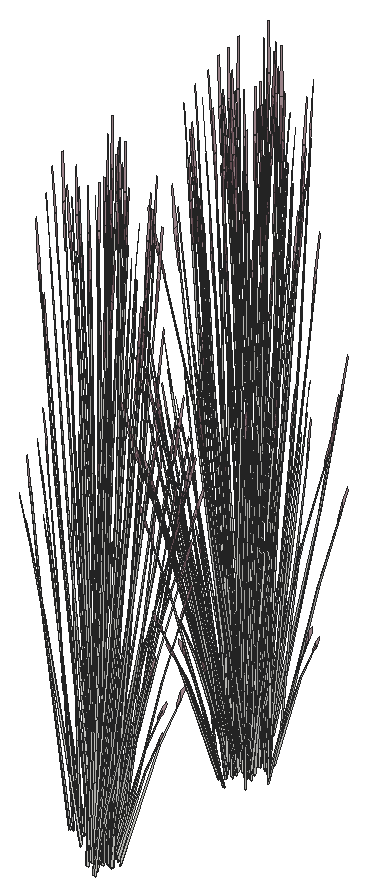
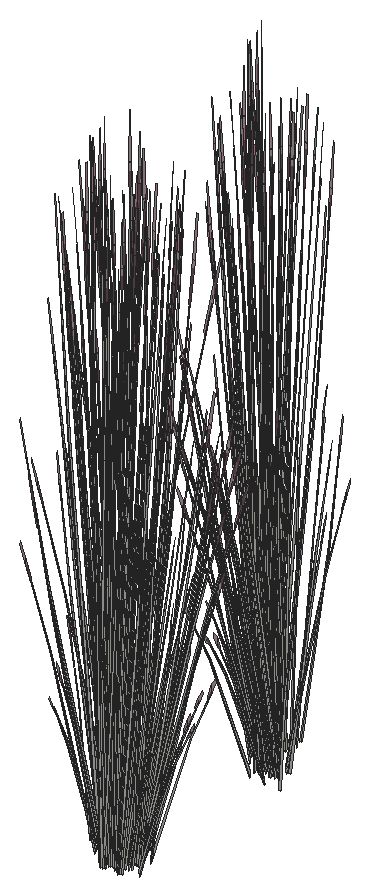
# SketchUp Ruby script. Lengths in inches.
U = 1.inch
M = Sketchup.active_model
def pt(a) = Geom::Point3d.new(a.map { |v| v * U })
def face(e, loops, mat)
  f = e.add_face(loops[0].map { |a| pt(a) })
  loops[1..].each { |l| e.add_face(l.map { |a| pt(a) }).erase! }
  f.material = f.back_material = mat if mat
  f
end
# faces: each face lists its corners as indices into pts; further lists are holes
def faces(e, pts, list, mat = nil) = list.each { |f| face(e, (f[0].is_a?(Array) ? f : [f]).map { |l| l.map { |i| pts[i] } }, mat) }
# xy, xz, yz: faces in a plane at the given z, y or x. An outline is a flat list of corners, or four numbers for a rectangle; further outlines are holes
def ring(l) = l.size == 4 ? [[l[0], l[1]], [l[2], l[1]], [l[2], l[3]], [l[0], l[3]]] : l.each_slice(2).to_a
def flat(e, list, mat, &to3) = list.each { |f| face(e, (f[0].is_a?(Array) ? f : [f]).map { |l| ring(l).map { |u, v| to3.(u, v) } }, mat) }
def xy(e, z, list, mat = nil) = flat(e, list, mat) { |x, y| [x, y, z] }
def xz(e, y, list, mat = nil) = flat(e, list, mat) { |x, z| [x, y, z] }
def yz(e, x, list, mat = nil) = flat(e, list, mat) { |y, z| [x, y, z] }
def lines(e, pts, list) = list.each { |a, b| e.add_line(pt(pts[a]), pt(pts[b])) }
# prism: a flat outline (further loops are holes) pulled along v
def prism(e, loops, v, mat = nil)
  f = face(e, loops, mat); d = Geom::Vector3d.new(v.map { |x| x * U })
  f.pushpull(f.normal.samedirection?(d) ? d.length : -d.length)
end
def box(e, o, s, mat = nil) = prism(e, [[o, [o[0] + s[0], o[1], o[2]], [o[0] + s[0], o[1] + s[1], o[2]], [o[0], o[1] + s[1], o[2]]]], [0, 0, s[2]], mat)
def at(x, y, z, deg = 0) = Geom::Transformation.translation(pt([x, y, z])) * Geom::Transformation.rotation(ORIGIN, Z_AXIS, deg.degrees)
def axes(o, x, y, z) = Geom::Transformation.new([*x, 0, *y, 0, *z, 0, *pt(o).to_a, 1])
def part(name) = M.definitions.add(name)
# library, detail: a bought-in or finely detailed component or shape, given as its bounding box
def library(name, o, s) = part(name).tap { |d| box(d.entities, o, s) }
def detail(e, o, s) = box(e.add_group.entities, o, s)
def put(e, d, t, mat = nil) = e.add_instance(d, t).tap { |i| i.material = mat if mat }
def group(e, t, mat = nil) = e.add_group.tap { |g| g.transformation = t; g.material = mat if mat }.entities
root = M.entities
M.materials.add("LightPink_Translucent").color = [144, 107, 117]
M.materials["LightPink_Translucent"].alpha = 0.75
c1 = part("blade")
p = [[2.15,0.21,22],[0,0.17,0],[0.09,0.45,0],[2.18,0.31,22],[2.29,0.31,22],[0.38,0.45,0],
  [2.48,0.24,33],[2.49,0.24,33],[2.48,0.22,33]]
faces(c1.entities,p,[[0,1,2,3],[4,5,2,3],[6,3,4,7],[8,0,3,6]])
c2 = part("seeds")
p = [[0.3,-0.1,1.38],[-0.01,-0.03,1.59],[-0.01,-0.03,0.03],[0.14,-0.07,-0.07],[0.29,-0.03,3],[0.15,0.01,3.11]]
faces(c2.entities,p,[[0,1,2,3],[1,0,4,5]],"LightPink_Translucent")
c3 = part("blade with seeds")
put(c3.entities,c1,at(0,0,0))
put(c3.entities,c2,axes([2.4,0.25,30.99],[1.5799,-0.05474,1.17369],[-0.12525,1.92788,0.29478],[-0.07173,-0.02425,1.56792]))
put(root,c3,axes([402.25,60.02,2.72],[-0.21202,-0.39143,0.44739],[0.32115,-0.27564,-0.21531],[0.06861,0.04843,1.43643]))
put(root,c3,axes([401.15,61.81,2.03],[-0.08291,-0.40636,-0.30978],[0.32928,-0.11539,0.30978],[-0.06638,-0.04686,1.38974]))
put(root,c3,axes([401.58,61.78,2.47],[0.37926,-0.12378,0.17642],[0.09365,0.46065,0.35086],[-0.03382,-0.06712,1.60407]))
put(root,c3,axes([402.36,60.04,2.67],[0.35635,-0.30962,-0.29095],[0.23697,0.43749,-0.50002],[0.08792,0.04443,1.59708]))
put(root,c3,axes([403.78,60.86,4.53],[0.29332,0.1301,-0.35414],[-0.08555,0.37955,0.4572],[0.11809,-0.0348,0.87481]))
put(root,c3,axes([401.0625,61.98,2.02],[-0.33032,-0.23318,-0.49651],[0.19744,-0.41812,0],[-0.07523,-0.05311,1.57504]))
put(root,c3,axes([403.26,59.22,2.02],[0.33032,0.23318,-0.49651],[-0.19744,0.41812,0],[0.07523,0.05311,1.57504]))
put(root,c3,axes([400.33,60.25,4.53],[-0.29332,-0.1301,-0.35414],[0.08555,-0.37955,0.4572],[-0.11809,0.0348,0.87481]))
put(root,c3,axes([402.63,60.55,2.21],[0.39487,0,0],[0,0.48281,0],[0,0,1.78407]))
put(root,c3,axes([401.96,61.16,2.67],[-0.35635,0.30962,-0.29095],[-0.23697,-0.43749,-0.50002],[-0.08792,-0.04443,1.59708]))
put(root,c3,axes([402.74,59.42,2.47],[-0.37926,0.12378,0.17642],[-0.09365,-0.46065,0.35086],[0.03382,0.06712,1.60407]))
put(root,c3,axes([402.98,60.39,3.875],[-0.14639,0.01056,1.71376],[0.09712,-0.45778,0.13857],[0.20862,0.02831,0.73262]))
put(root,c3,axes([403.17,59.39,2.03],[0.08291,0.40636,-0.30978],[-0.32928,0.11539,0.30978],[0.06638,0.04686,1.38974]))
put(root,c3,axes([402.5,60.3,2.38],[-0.44609,-0.09826,0.49198],[0.09078,-0.55493,0.19306],[0.06519,0.05359,1.70813]))
put(root,c3,axes([402.15,61.67,2.2],[-0.11516,-0.40207,0],[0.32884,-0.1408,0],[0,0,1.54371]))
put(root,c3,axes([401.93,61.29,2.62],[-0.06809,0.4162,0.1448],[-0.33266,-0.07225,-0.41347],[-0.06054,-0.04274,1.26744]))
put(root,c3,axes([402.58,61.62,2.18],[0.37054,-0.15823,-0.19198],[0.1302,0.45581,0.00008],[0.0409,-0.01749,1.73897]))
put(root,c3,axes([402.71,61.81,2.47],[0.10196,-0.46348,0.17642],[0.3731,0.13116,0.35086],[-0.06445,0.00226,1.60407]))
put(root,c3,axes([402.62,60.76,2.21],[0.24637,0.30123,0],[-0.24637,0.30123,0],[0,0,1.69266]))
put(root,c3,axes([401.22,60.19,3.34],[0.10032,-0.06746,1.77064],[0.0346,0.47103,0.13857],[-0.2173,0.0625,0.63284]))
put(root,c3,axes([403.29,60.625,2.47],[-0.2773,-0.3397,0.17642],[0.27945,-0.32949,0.35086],[-0.03063,0.06937,1.60407]))
put(root,c3,axes([402.78,60.11,2.06],[0.36714,0.07646,-0.62353],[-0.07747,0.47163,-0.16365],[0.10956,0.05715,1.37633]))
put(root,c3,axes([404.4,60.9375,2.77],[-0.21807,0.07699,1.1486],[0.10265,-0.31819,0.84392],[0.11568,0.02177,0.25299]))
put(root,c3,axes([402.07,61.86,2.2],[-0.35581,-0.20937,0],[0.17124,-0.43505,0],[0,0,1.62707]))
put(root,c3,axes([402.36,61.3,2.46],[-0.34464,-0.37536,-0.25192],[0.29,-0.42149,0.5513],[-0.0928,0.04391,1.68216]))
put(root,c3,axes([401.45,62.02,2.48],[0.33032,0.23318,0.49651],[-0.19744,0.41812,0],[-0.07523,-0.05311,1.57504]))
put(root,c3,axes([402.62,60.4,2.72],[0.17124,-0.42022,0.44739],[0.35581,0.20224,-0.21531],[0,0.09687,1.43643]))
put(root,c3,axes([402.55,60.64,2.29],[0,0.53934,-0.05637],[-0.44133,0,0],[0,0.01695,1.79368]))
put(root,c3,axes([400.53,60.45,4.68],[-0.09562,0.42421,-0.51099],[-0.32782,-0.1454,-0.3958],[-0.13199,0.0389,0.97773]))
put(root,c3,axes([402.58,60.26,2.21],[0.21202,0.39143,-0.44739],[-0.32115,0.27564,0.21531],[0.06861,0.04843,1.43643]))
put(root,c3,axes([404.02,61.92,3.93],[-0.06755,-0.39203,-0.03492],[0.31928,-0.09013,-0.15832],[0.06667,0.02485,0.52218]))
put(root,c3,axes([401.26,62.26,2.375],[-0.22066,0.46731,0],[-0.36918,-0.26061,-0.51607],[-0.08408,-0.05936,1.63711]))
put(root,c3,axes([403.52,60.64,2.48],[0,-0.46636,0.49651],[0.39487,0,0],[0,0.10622,1.57504]))
put(root,c3,axes([402.53,60.99,2.72],[0.38326,-0.02879,0.44739],[0.03466,0.47788,-0.21531],[-0.06861,0.04843,1.43643]))
put(root,c3,axes([402.77,60.5,2.62],[0.32884,-0.136,0.1448],[0.11516,0.38837,-0.41347],[0,0.08547,1.26744]))
put(root,c3,axes([402.1875,61.22,2.21],[-0.38326,0.02879,-0.44739],[-0.03466,-0.47788,0.21531],[-0.06861,0.04843,1.43643]))
put(root,c3,axes([403.99,61.45,2.59],[-0.085,-0.1147,1.43002],[0.1106,-0.37943,-0.30754],[0.17198,0.0514,0.61141]))
put(root,c3,axes([402.47,61.86,2.2],[0.35581,0.20937,0],[-0.17124,0.43505,0],[0,0,1.74954]))
put(root,c3,axes([402.61,62.33,2.19],[-0.21791,-0.46895,-0.05142],[0.36918,-0.26061,0.51607],[-0.09097,0.04465,1.6363]))
put(root,c3,axes([402.53,61.19,2.62],[0.26075,0.2802,0.1448],[-0.2175,0.31612,-0.41347],[-0.06054,0.04274,1.26744]))
put(root,c3,axes([400.52,60.67,3.875],[0.12246,-0.09864,1.71376],[0.1031,0.45582,0.13857],[-0.19225,0.10302,0.73262]))
put(root,c3,axes([403.21,61.68,4.98],[0.35281,0.01123,-0.71045],[-0.0237,0.47284,0.08574],[0.14947,0.0499,1.00501]))
put(root,c3,axes([402.8125,62.06,2.48],[0.33032,-0.23318,0.49651],[0.19744,0.41812,0],[-0.07523,0.05311,1.57504]))
put(root,c3,axes([402.34,61.6875,2.29],[0.15345,0.53576,-0.06012],[-0.43845,0.18773,0],[0.00536,0.01871,1.72173]))
put(root,c3,axes([402.51,62.27,2.03],[-0.32928,-0.11539,-0.30978],[0.08291,-0.40636,0.30978],[-0.06638,0.04686,1.38974]))
put(root,c3,axes([400.14,61.44,2.59],[0.12266,0.03828,1.43002],[0.07906,0.39104,-0.30754],[-0.16661,0.0732,0.61141]))
put(root,c3,axes([403.78,60.72,2.375],[0.44133,0,0],[0,0.52122,-0.51607],[0,0.11871,1.63711]))
put(root,c3,axes([403.61,60.99,2.2],[-0.44111,-0.00373,-0.04976],[0,-0.52122,0.49943],[-0.01386,0.11865,1.58352]))
put(root,c3,axes([402.65,60.53,2.67],[0.39748,0.22252,-0.29095],[-0.19139,0.46966,-0.50002],[0.01249,0.11531,1.59708]))
put(root,c3,axes([399.88,62.26,2.77],[0.14709,-0.21136,1.1486],[0.05804,0.3346,0.84392],[-0.1063,0.05991,0.25299]))
put(root,c3,axes([403.42,61.87,4.53],[0.20082,0.29199,-0.35414],[-0.2293,0.2764,0.4572],[0.1165,0.04206,0.87481]))
put(root,c3,axes([403.52,61.0625,2.03],[-0.24637,0.29097,-0.30978],[-0.24637,-0.29097,0.30978],[0,0.09372,1.38974]))
put(root,c3,axes([402.46,61.09,2.67],[0.04113,0.53214,-0.29095],[-0.42835,0.03218,-0.50002],[-0.07543,0.07088,1.59708]))
put(root,c3,axes([402.61,60.88,2.21],[-0.17124,0.42022,-0.44739],[-0.35581,-0.20224,0.21531],[0,0.09687,1.43643]))
put(root,c3,axes([400.43,61.35,4.53],[-0.30722,0.06665,-0.35414],[-0.08112,-0.381,0.4572],[-0.08804,0.10234,0.87481]))
put(root,c3,axes([402.2,61.5,2.06],[-0.23773,0.35053,-0.62353],[-0.29532,-0.31785,-0.16365],[-0.09526,0.08744,1.37633]))
put(root,c3,axes([402.62,62.09,2.33],[0.44186,0.15158,0.30756],[-0.11054,0.54181,-0.36492],[-0.07313,0.06781,1.64885]))
put(root,c3,axes([402.59,62.45,2.02],[-0.33032,0.23318,-0.49651],[-0.19744,-0.41812,0],[-0.07523,0.05311,1.57504]))
put(root,c3,axes([403.6875,61.07,2.02],[0,0.46636,-0.49651],[-0.39487,0,0],[0,0.10622,1.57504]))
put(root,c3,axes([402.7,61.125,3.875],[-0.1311,-0.08035,1.71376],[0.27131,-0.33708,0.13857],[0.16909,0.15206,0.73262]))
put(root,c3,axes([403.18,62.04,2.77],[-0.19872,-0.13409,1.1486],[0.2566,-0.13625,0.84392],[0.06921,0.11541,0.25299]))
put(root,c3,axes([400.97,60.97,3.875],[0.08815,-0.14329,1.71376],[0.22258,0.38678,0.13857],[-0.15267,0.17614,0.73262]))
put(root,c3,axes([400.6875,61.39,4.68],[0.09067,0.42583,-0.51099],[-0.34336,0.07449,-0.3958],[-0.0984,0.11438,0.97773]))
put(root,c3,axes([402.89,62.38,2.375],[0.22066,0.46731,0],[-0.36918,0.26061,-0.51607],[-0.08408,0.05936,1.63711]))
put(root,c3,axes([403.24,62.54,1.49],[0.02571,-0.06733,1.76342],[0.32373,-0.19829,-0.26939],[0.09815,0.10263,0.30037]))
put(root,c3,axes([402.7,60.53,2.84],[-0.00964,-0.43909,1.41272],[0.43635,0.11382,0.59816],[-0.1032,0.24027,1.3335]))
put(root,c3,axes([402.8125,61.01,2.09],[0.12941,0.42699,-0.69212],[-0.37279,0.15378,-0.18165],[0.0143,0.14459,1.52773]))
put(root,c3,axes([400.27,62.48,1.49],[0.04734,0.04659,1.76342],[0.08027,0.4317,-0.26939],[-0.10492,0.09206,0.30037]))
put(root,c3,axes([402.74,62.22,4.68],[0.34827,-0.11086,-0.51099],[0.06092,0.41983,-0.3958],[0.09354,0.12031,0.97773]))
put(root,c3,axes([403.22,62.65,2.67],[-0.22633,-0.01463,1.0506],[0.14947,-0.31064,0.58006],[0.08941,0.11036,0.8241]))
put(root,c3,axes([400.9,61.33,3.875],[0.06572,-0.16029,1.71376],[0.27569,0.33172,0.13857],[-0.12437,0.20675,0.73262]))
put(root,c3,axes([402.48,61.9,2.59],[0.00623,-0.15459,1.43002],[0.29764,-0.17268,-0.30754],[0.09188,0.18503,0.61141]))
put(root,c3,axes([400.98,62.23,4.53],[-0.23881,0.24554,-0.35414],[-0.22606,-0.28036,0.4572],[-0.0344,0.14245,0.87481]))
put(root,c3,axes([401.13,63.18,2.77],[-0.00913,-0.2773,1.1486],[0.22824,0.19778,0.84392],[-0.04489,0.13217,0.25299]))
put(root,c3,axes([401.73,62.52,1.49],[0.05712,-0.02538,1.76342],[0.34359,0.13968,-0.26939],[0.01005,0.15742,0.30037]))
put(root,c3,axes([401.21,62.11,5],[0.25266,0.31335,-0.5672],[-0.2669,0.27442,-0.43934],[-0.03844,0.15921,1.08528]))
put(root,c3,axes([400.9375,62.59,2.82],[0.32063,-0.08258,0.06507],[0.07371,0.33271,-0.86304],[-0.02033,0.16842,0.7736]))
put(root,c3,axes([401.96,62.42,4.68],[0.34695,0.11691,-0.51099],[-0.11892,0.40083,-0.3958],[0.03181,0.16138,0.97773]))
put(root,c3,axes([402.16,61.59,3.875],[-0.08068,-0.14973,1.71376],[0.3728,-0.12606,0.13857],[0.08426,0.23506,0.73262]))
put(root,c3,axes([401.8,62.66,4.53],[-0.1064,0.35863,-0.35414],[-0.31043,-0.1046,0.4572],[0.02846,0.14439,0.87481]))
put(root,c3,axes([401.13,61.97,5.34],[-0.00918,0.43138,-0.7886],[-0.38672,-0.02897,0.09517],[-0.04081,0.18275,1.11556]))
put(root,c3,axes([401.5,61.67,3.875],[-0.00864,-0.17899,1.71376],[0.37441,0.11874,0.13857],[-0.02316,0.25508,0.73262]))
put(root,c3,axes([401.84,62.34,4.98],[0.16845,0.3792,-0.71045],[-0.34676,0.21133,0.08574],[0.03939,0.18322,1.00501]))
put(root,c3,axes([400.86,62.9375,2.59],[0.11138,-0.07357,1.43002],[0.27499,0.22183,-0.30754],[-0.08185,0.19194,0.61141]))
put(root,c3,axes([401.01,62.58,3.36],[0.00775,-0.24075,1.54345],[0.34877,0.12716,0.21329],[-0.03022,0.25658,0.72882]))
put(root,c3,axes([401.27,77.76,3.875],[0.08068,0.14973,1.71376],[-0.3728,0.12606,0.13857],[-0.08426,-0.23506,0.73262]))
put(root,c3,axes([402.72,77.54,2.59],[-0.10032,0.0944,1.43002],[-0.30046,-0.16522,-0.30754],[0.05569,-0.20547,0.61141]))
put(root,c3,axes([402.27,77.87,4.98],[-0.16845,-0.3792,-0.71045],[0.34676,-0.21133,0.08574],[-0.03939,-0.18322,1.00501]))
put(root,c3,axes([401.17,77.36,2.59],[-0.02137,0.15256,1.43002],[-0.31245,0.12771,-0.30754],[-0.07303,-0.19719,0.61141]))
put(root,c3,axes([401.98,77.03,1.49],[-0.0592,0.0168,1.76342],[-0.32738,-0.18913,-0.26939],[0.00549,-0.15776,0.30037]))
put(root,c3,axes([402.97,78.24,4.98],[0.00918,-0.43138,-0.71045],[0.38672,0.02897,0.08574],[0.04081,-0.18275,1.00501]))
put(root,c3,axes([402.3,77.54,4.53],[0.1064,-0.35863,-0.35414],[0.31043,0.1046,0.4572],[-0.02846,-0.14439,0.87481]))
put(root,c3,axes([402.53,78.02,3.875],[-0.06572,0.16029,1.71376],[-0.27569,-0.33172,0.13857],[0.12437,-0.20675,0.73262]))
put(root,c3,axes([402.14,77.79,4.68],[-0.34695,-0.11691,-0.51099],[0.11892,-0.40083,-0.3958],[-0.03181,-0.16138,0.97773]))
put(root,c3,axes([402.35,76.79,2.77],[0.04528,0.27194,1.1486],[-0.25117,-0.15062,0.84392],[0.02703,-0.13924,0.25299]))
put(root,c3,axes([402.89,78.09,4.68],[-0.25266,-0.31335,-0.51099],[0.2669,-0.27442,-0.3958],[0.03844,-0.15921,0.97773]))
put(root,c3,axes([403.13,77.98,4.53],[0.23881,-0.24554,-0.35414],[0.22606,0.28036,0.4572],[0.0344,-0.14245,0.87481]))
put(root,c3,axes([401.0625,77.11,2.77],[0.18411,0.16231,1.1486],[-0.26813,0.09757,0.84392],[-0.05737,-0.12474,0.25299]))
put(root,c3,axes([401.51,77.97,4.98],[-0.30095,-0.22541,-0.71045],[0.21388,-0.395,0.08574],[-0.10904,-0.13459,1.00501]))
put(root,c3,axes([401.4,77.68,4.53],[-0.05451,-0.37564,-0.35414],[0.31161,-0.09919,0.4572],[-0.0837,-0.10765,0.87481]))
put(root,c3,axes([400.92,77.6,1.49],[-0.03419,0.06144,1.76342],[-0.3455,0.13246,-0.26939],[-0.08346,-0.12049,0.30037]))
put(root,c3,axes([401.49,79.29,2.1],[-0.14494,-0.47823,-0.69835],[0.41752,-0.17223,-0.18329],[-0.01602,-0.16194,1.54149]))
put(root,c3,axes([400.73,78.22,3.875],[0.1311,0.08035,1.71376],[-0.27131,0.33708,0.13857],[-0.16909,-0.15206,0.73262]))
put(root,c3,axes([403.43,77.83,1.49],[-0.05283,-0.03674,1.76342],[-0.13569,-0.41045,-0.26939],[0.09154,-0.11138,0.30037]))
put(root,c3,axes([401.37,77.99,4.68],[-0.34827,0.11086,-0.51099],[-0.06092,-0.41983,-0.3958],[-0.09354,-0.12031,0.97773]))
put(root,c3,axes([403.42,78.99,4.98],[0.18436,-0.36797,-0.71045],[0.32306,0.26151,0.08574],[0.11008,-0.13332,1.00501]))
put(root,c3,axes([401.43,77.92,2.375],[-0.22066,-0.46731,0],[0.36918,-0.26061,-0.51607],[0.08408,-0.05936,1.63711]))
put(root,c3,axes([403.41,78.82,4.68],[-0.09067,-0.42583,-0.51099],[0.34336,-0.07449,-0.3958],[0.0984,-0.11438,0.97773]))
put(root,c3,axes([401.92,77.35,2.13],[-0.2439,0.26754,-0.03893],[-0.22348,-0.29302,-0.17649],[-0.01573,-0.08303,0.58215]))
put(root,c3,axes([402.23,80.52,3.33],[0.305,0.18805,1.51261],[-0.29879,0.40513,0.59816],[-0.13384,-0.24012,1.26806]))
put(root,c3,axes([400.63,79.22,2.02],[0,-0.46636,-0.49651],[0.39487,0,0],[0,-0.10622,1.57504]))
put(root,c3,axes([401.73,77.84,2.02],[0.33032,-0.23318,-0.49651],[0.19744,0.41812,0],[0.07523,-0.05311,1.57504]))
put(root,c3,axes([403.69,78.65,2.59],[-0.12609,-0.01381,1.43002],[-0.12917,-0.37055,-0.30754],[0.1549,-0.10482,0.61141]))
put(root,c3,axes([402.12,78.8,2.06],[0.23773,-0.35053,-0.62353],[0.29532,0.31785,-0.16365],[0.09526,-0.08744,1.37633]))
put(root,c3,axes([403.84,77.97,2.77],[-0.11756,0.2374,1.1486],[-0.10105,-0.31895,0.84392],[0.09709,-0.07992,0.25299]))
put(root,c3,axes([403.67,78.86,4.53],[0.30722,-0.06665,-0.35414],[0.08112,0.381,0.4572],[0.08804,-0.10234,0.87481]))
put(root,c3,axes([401.71,79.41,2.21],[0.17124,-0.42022,-0.44739],[0.35581,0.20224,0.21531],[0,-0.09687,1.43643]))
put(root,c3,axes([400.68,78.34,4.53],[-0.20082,-0.29199,-0.35414],[0.2293,-0.2764,0.4572],[-0.1165,-0.04206,0.87481]))
put(root,c3,axes([401.86,79.21,2.67],[-0.04113,-0.53214,-0.29095],[0.42835,-0.03218,-0.50002],[0.07543,-0.07088,1.59708]))
put(root,c3,axes([400.8,79.23,2.03],[0.24637,-0.29097,-0.30978],[0.24637,0.29097,0.30978],[0,-0.09372,1.38974]))
put(root,c3,axes([400.7,77.84,2.13],[-0.10181,0.3808,-0.03893],[-0.31336,-0.11714,-0.17649],[-0.04758,-0.06228,0.58215]))
put(root,c3,axes([401.67,79.76,2.67],[-0.39748,-0.22252,-0.29095],[0.19139,-0.46966,-0.50002],[-0.01249,-0.11531,1.59708]))
put(root,c3,axes([400.53,79.58,2.375],[-0.44133,0,0],[0,-0.52122,-0.51607],[0,-0.11871,1.63711]))
put(root,c3,axes([400.61,78.65,2.59],[0.06891,0.12984,1.43002],[-0.15879,0.35293,-0.30754],[-0.16304,-0.08436,0.61141]))
put(root,c3,axes([401.81,78.03,2.03],[0.32928,0.11539,-0.30978],[-0.08291,0.40636,0.30978],[0.06638,-0.04686,1.38974]))
put(root,c3,axes([400.89,78.53,4.98],[-0.35281,-0.01123,-0.71045],[0.0237,-0.47284,0.08574],[-0.14947,-0.0499,1.00501]))
put(root,c3,axes([400.875,79.44,2.33],[-0.32829,0.39208,0.30756],[-0.32849,-0.38796,-0.36492],[-0.01146,-0.11134,1.64885]))
put(root,c3,axes([401.92,79.625,2.43],[0.39767,0.22603,0.24065],[-0.19139,0.46966,0.50002],[0,-0.10827,1.60543]))
put(root,c3,axes([401.77,80.26,2.4375],[0.09355,-0.55261,-0.23429],[0.44354,0.09633,0.51271],[-0.0775,-0.07631,1.5644]))
put(root,c3,axes([400.78,78.63,4.68],[-0.25628,0.30892,-0.51099],[-0.22444,-0.32634,-0.3958],[-0.13021,-0.047,0.97773]))
put(root,c3,axes([400.2,79.04,2.77],[0.22533,-0.03337,1.1486],[-0.14293,0.29403,0.84392],[-0.11135,-0.04411,0.25299]))
put(root,c3,axes([401.79,79.31,2.72],[-0.38326,0.02879,0.44739],[-0.03466,-0.47788,-0.21531],[0.06861,-0.04843,1.43643]))
put(root,c3,axes([400.8,79.66,2.48],[0,0.46636,0.49651],[-0.39487,0,0],[0,-0.10622,1.57504]))
put(root,c3,axes([403.57,79.76,4.68],[0.09562,-0.42421,-0.51099],[0.32782,0.1454,-0.3958],[0.13199,-0.0389,0.97773]))
put(root,c3,axes([403.06,78.03,2.375],[0.22066,-0.46731,0],[0.36918,0.26061,-0.51607],[0.08408,0.05936,1.63711]))
put(root,c3,axes([400.46,78.96,3.875],[0.14639,-0.01056,1.71376],[-0.09712,0.45778,0.13857],[-0.20862,-0.02831,0.73262]))
put(root,c3,axes([401.73,80.03,2.21],[-0.21202,-0.39143,-0.44739],[0.32115,-0.27564,0.21531],[-0.06861,-0.04843,1.43643]))
put(root,c3,axes([401.78,79.48,2.36],[0.15345,0.52148,0.45755],[-0.43845,0.18134,0.17955],[0.00536,-0.09582,1.58856]))
put(root,c3,axes([403.92,79.88,1.98],[-0.22732,0.05597,1.41583],[-0.03618,-0.44548,0.08104],[0.15921,-0.06743,0.80566]))
put(root,c3,axes([404.34,79.49,2.26],[-0.21881,-0.29821,-0.06488],[0.23965,-0.27324,-0.29416],[0.0679,-0.01924,0.97024]))
put(root,c3,axes([401.7,79.89,2.72],[-0.17124,0.42022,0.44739],[-0.35581,-0.20224,-0.21531],[0,-0.09687,1.43643]))
put(root,c3,axes([402.33,79.53,2.21],[0,-0.53961,0],[0.44133,0,0],[0,0,1.79456]))
put(root,c3,axes([402.87,78.28,2.48],[-0.33032,-0.23318,0.49651],[0.19744,-0.41812,0],[0.07523,0.05311,1.57504]))
put(root,c3,axes([403.51,79.92,4.98],[0.31014,-0.20596,-0.71045],[0.17284,0.42397,0.08574],[0.14985,-0.04816,1.00501]))
put(root,c3,axes([401.54,80.18,2.06],[-0.36714,-0.07646,-0.62353],[0.07747,-0.47163,-0.16365],[-0.10956,-0.05715,1.37633]))
put(root,c3,axes([402.12,79.19,2.36],[-0.29264,0.42323,0.45755],[-0.34767,-0.3736,0.17955],[0.07055,-0.04224,1.58856]))
put(root,c3,axes([402.44,79.94,2.3],[-0.32829,-0.4014,-0.06131],[0.32849,-0.40164,0],[-0.01146,-0.01402,1.75571]))
put(root,c3,axes([401.61,78.49,2.47],[-0.10196,0.46348,0.17642],[-0.3731,-0.13116,0.35086],[0.06445,-0.00226,1.60407]))
put(root,c3,axes([401.46,78.86,1.59],[-0.3474,0.18671,1.28929],[-0.11057,-0.53572,0.50096],[0.21332,0.00891,1.46642]))
put(root,c3,axes([402.39,79,2.62],[0.06809,-0.4162,0.1448],[0.33266,0.07225,-0.41347],[0.06054,0.04274,1.26744]))
put(root,c3,axes([401.82,79.99,2.36],[0.44609,0.09826,0.45755],[-0.09078,0.55493,0.17955],[-0.06519,-0.05359,1.58856]))
put(root,c3,axes([404.17,79.59,1.49],[-0.01845,-0.0708,1.76342],[0.12793,-0.41416,-0.26939],[0.12905,-0.00596,0.30037]))
put(root,c3,axes([400.36,79.52,1.49],[0.00895,0.0735,1.76342],[-0.18044,0.38382,-0.26939],[-0.12817,-0.01935,0.30037]))
put(root,c3,axes([402.25,79.11,2.72],[-0.21202,-0.39143,0.44739],[0.32115,-0.27564,-0.21531],[0.06861,0.04843,1.43643]))
put(root,c3,axes([401.15,80.9,2.03],[-0.08291,-0.40636,-0.30978],[0.32928,-0.11539,0.30978],[-0.06638,-0.04686,1.38974]))
put(root,c3,axes([401.58,80.88,2.47],[0.37926,-0.12378,0.17642],[0.09365,0.46065,0.35086],[-0.03382,-0.06712,1.60407]))
put(root,c3,axes([402.36,79.14,2.67],[0.35635,-0.30962,-0.29095],[0.23697,0.43749,-0.50002],[0.08792,0.04443,1.59708]))
put(root,c3,axes([403.78,79.95,4.53],[0.29332,0.1301,-0.35414],[-0.08555,0.37955,0.4572],[0.11809,-0.0348,0.87481]))
put(root,c3,axes([401.0625,81.08,2.02],[-0.33032,-0.23318,-0.49651],[0.19744,-0.41812,0],[-0.07523,-0.05311,1.57504]))
put(root,c3,axes([403.26,78.32,2.02],[0.33032,0.23318,-0.49651],[-0.19744,0.41812,0],[0.07523,0.05311,1.57504]))
put(root,c3,axes([400.33,79.35,4.53],[-0.29332,-0.1301,-0.35414],[0.08555,-0.37955,0.4572],[-0.11809,0.0348,0.87481]))
put(root,c3,axes([402.63,79.65,2.21],[0.39487,0,0],[0,0.48281,0],[0,0,1.78407]))
put(root,c3,axes([401.96,80.25,2.67],[-0.35635,0.30962,-0.29095],[-0.23697,-0.43749,-0.50002],[-0.08792,-0.04443,1.59708]))
put(root,c3,axes([402.74,78.51,2.47],[-0.37926,0.12378,0.17642],[-0.09365,-0.46065,0.35086],[0.03382,0.06712,1.60407]))
put(root,c3,axes([402.98,79.49,3.875],[-0.14639,0.01056,1.71376],[0.09712,-0.45778,0.13857],[0.20862,0.02831,0.73262]))
put(root,c3,axes([403.17,78.49,2.03],[0.08291,0.40636,-0.30978],[-0.32928,0.11539,0.30978],[0.06638,0.04686,1.38974]))
put(root,c3,axes([402.5,79.4,2.38],[-0.44609,-0.09826,0.49198],[0.09078,-0.55493,0.19306],[0.06519,0.05359,1.70813]))
put(root,c3,axes([402.15,80.77,2.2],[-0.11516,-0.40207,0],[0.32884,-0.1408,0],[0,0,1.54371]))
put(root,c3,axes([401.93,80.39,2.62],[-0.06809,0.4162,0.1448],[-0.33266,-0.07225,-0.41347],[-0.06054,-0.04274,1.26744]))
put(root,c3,axes([402.58,80.71,2.18],[0.37054,-0.15823,-0.19198],[0.1302,0.45581,0.00008],[0.0409,-0.01749,1.73897]))
put(root,c3,axes([402.71,80.9,2.47],[0.10196,-0.46348,0.17642],[0.3731,0.13116,0.35086],[-0.06445,0.00226,1.60407]))
put(root,c3,axes([402.62,79.85,2.21],[0.24637,0.30123,0],[-0.24637,0.30123,0],[0,0,1.69266]))
put(root,c3,axes([401.22,79.29,3.34],[0.10032,-0.06746,1.77064],[0.0346,0.47103,0.13857],[-0.2173,0.0625,0.63284]))
put(root,c3,axes([403.29,79.72,2.47],[-0.2773,-0.3397,0.17642],[0.27945,-0.32949,0.35086],[-0.03063,0.06937,1.60407]))
put(root,c3,axes([402.78,79.21,2.06],[0.36714,0.07646,-0.62353],[-0.07747,0.47163,-0.16365],[0.10956,0.05715,1.37633]))
put(root,c3,axes([404.4,80.03,2.77],[-0.21807,0.07699,1.1486],[0.10265,-0.31819,0.84392],[0.11568,0.02177,0.25299]))
put(root,c3,axes([402.07,80.95,2.2],[-0.35581,-0.20937,0],[0.17124,-0.43505,0],[0,0,1.62707]))
put(root,c3,axes([402.36,80.39,2.46],[-0.34464,-0.37536,-0.25192],[0.29,-0.42149,0.5513],[-0.0928,0.04391,1.68216]))
put(root,c3,axes([401.45,81.11,2.48],[0.33032,0.23318,0.49651],[-0.19744,0.41812,0],[-0.07523,-0.05311,1.57504]))
put(root,c3,axes([402.62,79.5,2.72],[0.17124,-0.42022,0.44739],[0.35581,0.20224,-0.21531],[0,0.09687,1.43643]))
put(root,c3,axes([402.55,79.74,2.29],[0,0.53934,-0.05637],[-0.44133,0,0],[0,0.01695,1.79368]))
put(root,c3,axes([400.53,79.54,4.68],[-0.09562,0.42421,-0.51099],[-0.32782,-0.1454,-0.3958],[-0.13199,0.0389,0.97773]))
put(root,c3,axes([402.58,79.36,2.21],[0.21202,0.39143,-0.44739],[-0.32115,0.27564,0.21531],[0.06861,0.04843,1.43643]))
put(root,c3,axes([404.02,81.01,3.93],[-0.06755,-0.39203,-0.03492],[0.31928,-0.09013,-0.15832],[0.06667,0.02485,0.52218]))
put(root,c3,axes([401.26,81.36,2.375],[-0.22066,0.46731,0],[-0.36918,-0.26061,-0.51607],[-0.08408,-0.05936,1.63711]))
put(root,c3,axes([403.52,79.73,2.48],[0,-0.46636,0.49651],[0.39487,0,0],[0,0.10622,1.57504]))
put(root,c3,axes([402.53,80.08,2.72],[0.38326,-0.02879,0.44739],[0.03466,0.47788,-0.21531],[-0.06861,0.04843,1.43643]))
put(root,c3,axes([402.77,79.6,2.62],[0.32884,-0.136,0.1448],[0.11516,0.38837,-0.41347],[0,0.08547,1.26744]))
put(root,c3,axes([402.1875,80.31,2.21],[-0.38326,0.02879,-0.44739],[-0.03466,-0.47788,0.21531],[-0.06861,0.04843,1.43643]))
put(root,c3,axes([403.99,80.54,2.59],[-0.085,-0.1147,1.43002],[0.1106,-0.37943,-0.30754],[0.17198,0.0514,0.61141]))
put(root,c3,axes([402.47,80.96,2.2],[0.35581,0.20937,0],[-0.17124,0.43505,0],[0,0,1.74954]))
put(root,c3,axes([402.61,81.42,2.19],[-0.21791,-0.46895,-0.05142],[0.36918,-0.26061,0.51607],[-0.09097,0.04465,1.6363]))
put(root,c3,axes([402.53,80.29,2.62],[0.26075,0.2802,0.1448],[-0.2175,0.31612,-0.41347],[-0.06054,0.04274,1.26744]))
put(root,c3,axes([400.52,79.76,3.875],[0.12246,-0.09864,1.71376],[0.1031,0.45582,0.13857],[-0.19225,0.10302,0.73262]))
put(root,c3,axes([403.21,80.77,4.98],[0.35281,0.01123,-0.71045],[-0.0237,0.47284,0.08574],[0.14947,0.0499,1.00501]))
put(root,c3,axes([402.8125,81.15,2.48],[0.33032,-0.23318,0.49651],[0.19744,0.41812,0],[-0.07523,0.05311,1.57504]))
put(root,c3,axes([402.34,80.78,2.29],[0.15345,0.53576,-0.06012],[-0.43845,0.18773,0],[0.00536,0.01871,1.72173]))
put(root,c3,axes([402.51,81.36,2.03],[-0.32928,-0.11539,-0.30978],[0.08291,-0.40636,0.30978],[-0.06638,0.04686,1.38974]))
put(root,c3,axes([400.14,80.54,2.59],[0.12266,0.03828,1.43002],[0.07906,0.39104,-0.30754],[-0.16661,0.0732,0.61141]))
put(root,c3,axes([403.78,79.8125,2.375],[0.44133,0,0],[0,0.52122,-0.51607],[0,0.11871,1.63711]))
put(root,c3,axes([403.61,80.08,2.2],[-0.44111,-0.00373,-0.04976],[0,-0.52122,0.49943],[-0.01386,0.11865,1.58352]))
put(root,c3,axes([402.65,79.63,2.67],[0.39748,0.22252,-0.29095],[-0.19139,0.46966,-0.50002],[0.01249,0.11531,1.59708]))
put(root,c3,axes([399.88,81.36,2.77],[0.14709,-0.21136,1.1486],[0.05804,0.3346,0.84392],[-0.1063,0.05991,0.25299]))
put(root,c3,axes([403.42,80.97,4.53],[0.20082,0.29199,-0.35414],[-0.2293,0.2764,0.4572],[0.1165,0.04206,0.87481]))
put(root,c3,axes([403.52,80.16,2.03],[-0.24637,0.29097,-0.30978],[-0.24637,-0.29097,0.30978],[0,0.09372,1.38974]))
put(root,c3,axes([402.46,80.19,2.67],[0.04113,0.53214,-0.29095],[-0.42835,0.03218,-0.50002],[-0.07543,0.07088,1.59708]))
put(root,c3,axes([402.61,79.98,2.21],[-0.17124,0.42022,-0.44739],[-0.35581,-0.20224,0.21531],[0,0.09687,1.43643]))
put(root,c3,axes([400.43,80.44,4.53],[-0.30722,0.06665,-0.35414],[-0.08112,-0.381,0.4572],[-0.08804,0.10234,0.87481]))
put(root,c3,axes([402.2,80.59,2.06],[-0.23773,0.35053,-0.62353],[-0.29532,-0.31785,-0.16365],[-0.09526,0.08744,1.37633]))
put(root,c3,axes([402.62,81.18,2.33],[0.44186,0.15158,0.30756],[-0.11054,0.54181,-0.36492],[-0.07313,0.06781,1.64885]))
